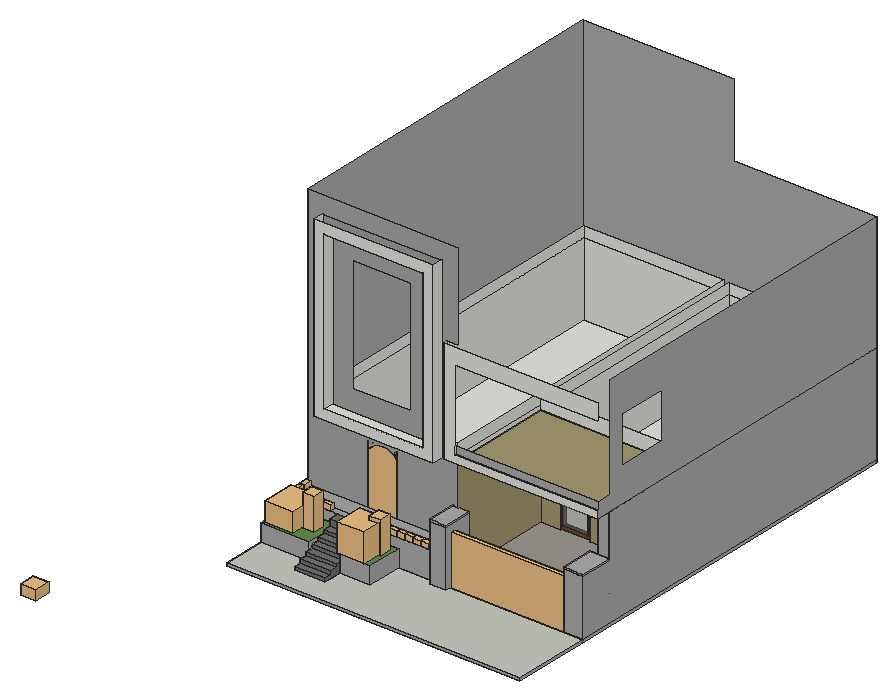
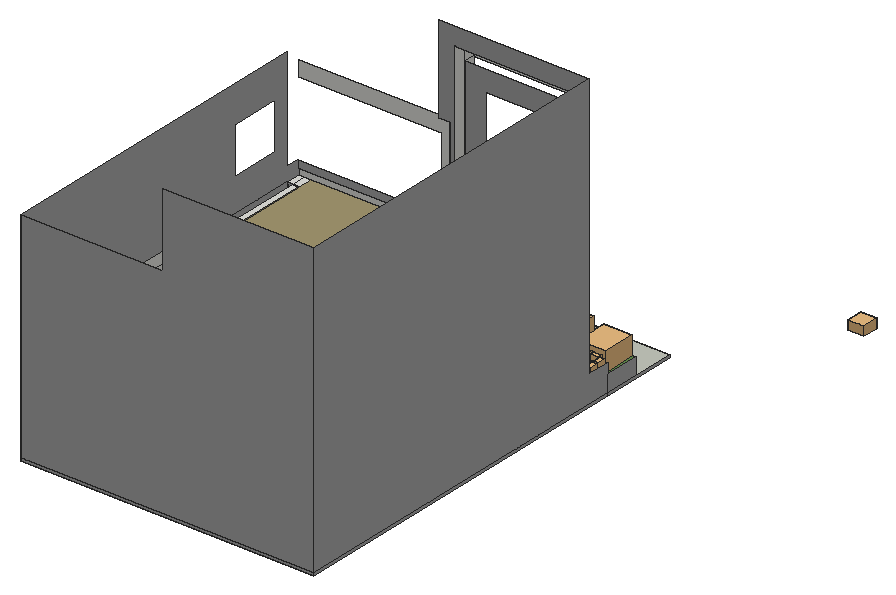
# SketchUp Ruby script. Lengths in inches.
U = 1.inch
M = Sketchup.active_model
def pt(a) = Geom::Point3d.new(a.map { |v| v * U })
def face(e, loops, mat)
  f = e.add_face(loops[0].map { |a| pt(a) })
  loops[1..].each { |l| e.add_face(l.map { |a| pt(a) }).erase! }
  f.material = f.back_material = mat if mat
  f
end
# faces: each face lists its corners as indices into pts; further lists are holes
def faces(e, pts, list, mat = nil) = list.each { |f| face(e, (f[0].is_a?(Array) ? f : [f]).map { |l| l.map { |i| pts[i] } }, mat) }
# xy, xz, yz: faces in a plane at the given z, y or x. An outline is a flat list of corners, or four numbers for a rectangle; further outlines are holes
def ring(l) = l.size == 4 ? [[l[0], l[1]], [l[2], l[1]], [l[2], l[3]], [l[0], l[3]]] : l.each_slice(2).to_a
def flat(e, list, mat, &to3) = list.each { |f| face(e, (f[0].is_a?(Array) ? f : [f]).map { |l| ring(l).map { |u, v| to3.(u, v) } }, mat) }
def xy(e, z, list, mat = nil) = flat(e, list, mat) { |x, y| [x, y, z] }
def xz(e, y, list, mat = nil) = flat(e, list, mat) { |x, z| [x, y, z] }
def yz(e, x, list, mat = nil) = flat(e, list, mat) { |y, z| [x, y, z] }
def lines(e, pts, list) = list.each { |a, b| e.add_line(pt(pts[a]), pt(pts[b])) }
# prism: a flat outline (further loops are holes) pulled along v
def prism(e, loops, v, mat = nil)
  f = face(e, loops, mat); d = Geom::Vector3d.new(v.map { |x| x * U })
  f.pushpull(f.normal.samedirection?(d) ? d.length : -d.length)
end
def box(e, o, s, mat = nil) = prism(e, [[o, [o[0] + s[0], o[1], o[2]], [o[0] + s[0], o[1] + s[1], o[2]], [o[0], o[1] + s[1], o[2]]]], [0, 0, s[2]], mat)
def at(x, y, z, deg = 0) = Geom::Transformation.translation(pt([x, y, z])) * Geom::Transformation.rotation(ORIGIN, Z_AXIS, deg.degrees)
def axes(o, x, y, z) = Geom::Transformation.new([*x, 0, *y, 0, *z, 0, *pt(o).to_a, 1])
def part(name) = M.definitions.add(name)
# library, detail: a bought-in or finely detailed component or shape, given as its bounding box
def library(name, o, s) = part(name).tap { |d| box(d.entities, o, s) }
def detail(e, o, s) = box(e.add_group.entities, o, s)
def put(e, d, t, mat = nil) = e.add_instance(d, t).tap { |i| i.material = mat if mat }
def group(e, t, mat = nil) = e.add_group.tap { |g| g.transformation = t; g.material = mat if mat }.entities
root = M.entities
M.materials.add("[Color M03]").color = [170, 170, 170]
M.materials.add("[Color M05]").color = [114, 114, 114]
M.materials.add("[Granite Tile]").color = [155, 148, 143]
M.materials.add("[Pavers with Grass Herringbone]").color = [197, 201, 190]
M.materials.add("[Stone Vein Gray]").color = [166, 165, 165]
M.materials.add("[Translucent Glass Gray]").color = [128, 128, 128]
M.materials["[Translucent Glass Gray]"].alpha = 0.5
M.materials.add("[Vegetation Grass Artificial]").color = [98, 140, 74]
M.materials.add("[Wood Lumber ButtJoined]").color = [164, 152, 112]
M.materials.add("[Wood Veneer 01]").color = [120, 70, 37]
c1 = library("Plant flower\#1",[15.36,-73.48,0],[25.38,25.65,15.83])
c2 = library("Group\#5",[0,0,0],[194.4375,4,109.5625])
c3 = library("Potted tree",[0,0,0],[18.46,18.88,52.55])
c4 = library("Group3\#1",[-239.85,50.56,0],[44.98,46.36,46.21])
c5 = library("Philodendron 3D",[-30.19,-30.88,0],[62.33,72.62,41.59])
c6 = library("VASINHOS CONCRETO COM SUCULENTAS",[7.69,5.35,0],[7.57,13.06,8.42])
c7 = part("Group\#1")
xy(c7.entities,0,[[0,0,48,9]],"[Wood Veneer 01]")
xy(c7.entities,3.71,[[3.71,0,21.93,9],[26.34,0,44.29,9]],"[Wood Veneer 01]")
xy(c7.entities,80.29,[[3.71,0,21.93,9],[26.34,0,44.29,9]],"[Wood Veneer 01]")
xy(c7.entities,84,[[0,0,48,9]],"[Wood Veneer 01]")
xz(c7.entities,0,[[3.71,3.71,21.93,80.29],[26.34,3.71,44.29,80.29]],"[Translucent Glass Gray]")
xz(c7.entities,0,[[[0,0,48,84],[3.71,3.71,21.93,80.29],[26.34,3.71,44.29,80.29]]],"[Wood Veneer 01]")
xz(c7.entities,9,[[[0,0,48,84],[3.71,3.71,44.29,80.29]],[21.93,3.71,26.34,80.29]],"[Wood Veneer 01]")
yz(c7.entities,0,[[0,0,9,84]],"[Wood Veneer 01]")
yz(c7.entities,3.71,[[0,3.71,9,80.29]],"[Wood Veneer 01]")
yz(c7.entities,21.93,[[0,3.71,9,80.29]],"[Wood Veneer 01]")
yz(c7.entities,26.34,[[0,3.71,9,80.29]],"[Wood Veneer 01]")
yz(c7.entities,44.29,[[0,3.71,9,80.29]],"[Wood Veneer 01]")
yz(c7.entities,48,[[0,0,9,84]],"[Wood Veneer 01]")
xy(root,0,[[4.125,0,484.125,127.875],[4.125,127.875,484.125,727.875]])
xy(root,4,[[83.39,39.19,132.89,51.19],[83.39,51.19,132.89,127.875],[4.125,69.64,83.39,127.875],[4.125,127.875,267.625,127.875,267.625,136.875,484.125,136.875,484.125,727.875,4.125,727.875],[267.625,127.875,475.125,136.875],
  [475.125,127.875,484.125,128.8125],[475.125,128.8125,484.125,136.875]])
xy(root,4,[[4.125,0,484.125,0,484.125,127.875,182.58,127.875,182.58,69.5625,132.89,69.5625,132.89,39.19,83.39,39.19,83.39,69.64,4.125,69.64]],"[Pavers with Grass Herringbone]")
xy(root,4.25,[[241.5,119.1875,267.625,127.875],[452.625,128.8125,475.125,136.875]])
xy(root,4.25,[[267.625,136.875,452.625,136.875,452.625,182.19,465.0625,182.19,465.0625,333.375,331.47,333.375,331.47,339.375,283.47,339.375,283.47,333.375,250.5,333.375,250.5,165.13,267.625,165.13]],"[Granite Tile]")
xy(root,9.5625,[[83.39,39.19,132.89,51.19]],"[Color M05]")
xy(root,15.125,[[83.39,51.19,132.89,63.19]],"[Color M05]")
xy(root,20.6875,[[83.39,63.19,132.89,75.19]],"[Color M05]")
xy(root,26.25,[[83.39,75.19,132.89,87.19]],"[Color M05]")
xy(root,31.8125,[[83.39,87.19,132.89,99.19]],"[Color M05]")
xy(root,31.8125,[[132.89,69.5625,182.58,127.875],[4.125,69.64,83.39,127.875]],"[Vegetation Grass Artificial]")
xy(root,37.375,[[83.39,99.19,132.89,111.19]],"[Color M05]")
xy(root,48,[[13.125,174.8125,241.5,718.875]])
xy(root,48,[[83.39,111.19,132.89,127.875]],"[Color M05]")
xy(root,48,[[4.125,127.875,241.5,127.875,241.5,136.875,13.125,136.875,13.125,165.13,4.125,165.13],[13.125,136.875,241.5,136.875,241.5,165.13,150.96,165.13,150.96,174.8125,102.96,174.8125,102.96,165.13,13.125,165.13]],"[Stone Vein Gray]")
xy(root,55.42,[[383.13,333.375,437.25,339.375]])
xy(root,96,[[452.625,128.8125,484.125,182.19]])
xy(root,99,[[452.625,128.8125,484.125,182.19]],"[Color M03]")
xy(root,99.3125,[[241.5,119.1875,267.625,165.13]],"[Color M03]")
xy(root,111.75,[[283.47,333.375,331.47,339.375]])
xy(root,119.86,[[383.13,333.375,437.25,339.375]])
xy(root,162.49,[[28.46,148.38,223.09,165.13]])
xy(root,168,[[232.4375,157.82,250.5,165.13],[465.0625,157.82,475.125,182.19],[475.125,157.82,484.125,182.19],[465.0625,182.19,475.125,333.375],[483.8125,182.19,484.125,727.875]])
xy(root,168,[[250.5,157.82,465.0625,333.375]],"[Wood Lumber ButtJoined]")
xy(root,178.89,[[44.86,148.38,206.69,165.13]])
xy(root,179.17,[[250.29,157.82,484.125,161.01]])
xz(root,0,[[4.125,0,484.125,4]],"[Color M03]")
xz(root,39.19,[[83.39,4,132.89,9.5625]],"[Color M05]")
xz(root,51.19,[[83.39,9.5625,132.89,15.125]],"[Color M05]")
xz(root,63.19,[[83.39,15.125,132.89,20.6875]],"[Color M05]")
xz(root,69.5625,[[132.89,4,182.58,31.8125]],"[Color M03]")
xz(root,69.64,[[4.125,4,83.39,31.8125]],"[Color M03]")
xz(root,75.19,[[83.39,20.6875,132.89,26.25]],"[Color M05]")
xz(root,87.19,[[83.39,26.25,132.89,31.8125]],"[Color M05]")
xz(root,99.19,[[83.39,31.8125,132.89,37.375]],"[Color M05]")
xz(root,111.19,[[83.39,37.375,132.89,48]],"[Color M05]")
xz(root,119.1875,[[241.5,4.25,267.625,96],[241.5,96,267.625,99.3125]],"[Color M03]")
xz(root,127.875,[[4.125,0,484.125,4],[4.125,4,83.39,31.8125],[83.39,4,132.89,37.375],[132.89,4,182.58,31.8125]])
xz(root,127.875,[[182.58,4,267.625,4,267.625,4.25,241.5,4.25,241.5,48,132.89,48,132.89,31.8125,182.58,31.8125],[4.125,31.8125,83.39,48]],"[Color M03]")
xz(root,128.8125,[[475.125,4,484.125,4,484.125,96,452.625,96,452.625,4.25,475.125,4.25],[452.625,96,484.125,99]],"[Color M03]")
xz(root,136.875,[[267.625,4,475.125,4.25]])
xz(root,148.38,[[[28.46,162.49,223.09,452.06],[44.86,178.89,206.69,435.66]]])
xz(root,157.82,[[232.4375,168,484.125,168,484.125,179.17,250.29,179.17,250.5,192,250.5,312,484.125,312,484.125,337.3125,232.4375,337.3125]])
xz(root,161.01,[[250.29,179.17,484.125,179.17,484.125,192,250.5,192]],"[Color M03]")
xz(root,165.13,[[250.5,4.25,267.625,96],[241.5,96,250.5,99.3125],[250.5,96,267.625,99.3125]])
xz(root,165.13,[[[4.125,48,102.96,48,102.96,132,105.82,135.82,109.27,139.1,113.24,141.76,117.59,143.72,122.2,144.91,126.96,145.3125,131.71,144.91,136.33,143.72,140.68,141.76,144.64,139.1,148.1,135.82,150.96,132,150.96,48,241.5,48,241.5,99.3125,250.5,99.3125,250.5,168,232.4375,168,232.4375,337.3125,250.5,337.3125,250.5,480,4.125,480],[28.46,162.49,223.09,452.06]],[[44.86,178.89,206.69,435.66],[78.82,212.85,172.73,401.7]]],"[Stone Vein Gray]")
xz(root,174.8125,[[13.125,48,13.125,186,241.5,186,241.5,48,150.96,48,150.96,132,148.1,135.82,144.64,139.1,140.68,141.76,136.33,143.72,131.71,144.91,126.96,145.3125,122.2,144.91,117.59,143.72,113.24,141.76,109.27,139.1,105.82,135.82,102.96,132,102.96,48]])
xz(root,182.19,[[452.625,4.25,465.0625,48],[452.625,48,465.0625,96],[452.625,96,465.0625,99],[465.0625,96,483.8125,99],[483.8125,96,484.125,99],
  [483.8125,99,484.125,168]])
xz(root,182.19,[[465.0625,99,483.8125,168]],"[Color M03]")
xz(root,333.375,[[250.5,168,475.125,192]])
xz(root,333.375,[[[250.5,4.25,283.47,4.25,283.47,111.75,331.47,111.75,331.47,4.25,465.0625,4.25,465.0625,168,250.5,168],[383.13,55.42,437.25,119.86]]],"[Wood Lumber ButtJoined]")
xz(root,339.375,[[283.47,4.25,331.47,6.1875],[[250.5,48,250.5,168,475.125,168,475.125,48,331.47,48,331.47,111.75,283.47,111.75,283.47,48],[383.13,55.42,437.25,119.86]],[250.5,168,475.125,186]])
xz(root,718.875,[[13.125,48,241.5,168],[250.5,48,475.125,168],[13.125,168,241.5,186],[250.5,168,475.125,186]])
xz(root,727.875,[[483.8125,48,484.125,168]])
xz(root,727.875,[[4.125,0,484.125,4],[4.125,4,4.125,480,250.5,480,250.5,360,484.125,360,484.125,168,483.8125,168,483.8125,48,484.125,48,484.125,4]],"[Color M03]")
yz(root,4.125,[[0,0,127.875,4],[127.875,0,727.875,4],[69.64,4,127.875,31.8125],[127.875,4,127.875,48,165.13,48,165.13,480,727.875,480,727.875,4]],"[Color M03]")
yz(root,13.125,[[174.8125,48,718.875,168],[174.8125,168,718.875,186]])
yz(root,28.46,[[148.38,162.49,165.13,452.06]])
yz(root,44.86,[[148.38,178.89,165.13,435.66]])
yz(root,83.39,[[69.64,4,69.64,20.6875,75.19,20.6875,75.19,26.25,87.19,26.25,87.19,31.8125,127.875,31.8125,127.875,4]])
yz(root,83.39,[[69.64,20.6875,75.19,20.6875,75.19,26.25,87.19,26.25,87.19,31.8125,69.64,31.8125]],"[Color M03]")
yz(root,83.39,[[39.19,4,39.19,9.5625,51.19,9.5625,51.19,15.125,63.19,15.125,63.19,20.6875,69.64,20.6875,69.64,4],[99.19,31.8125,99.19,37.375,111.19,37.375,111.19,48,127.875,48,127.875,31.8125]],"[Color M05]")
yz(root,102.96,[[165.13,48,174.8125,132]])
yz(root,132.89,[[69.5625,4,127.875,4,127.875,31.8125,87.19,31.8125,87.19,26.25,75.19,26.25,75.19,20.6875,69.5625,20.6875]])
yz(root,132.89,[[69.5625,20.6875,69.5625,31.8125,87.19,31.8125,87.19,26.25,75.19,26.25,75.19,20.6875]],"[Color M03]")
yz(root,132.89,[[39.19,4,69.5625,4,69.5625,20.6875,63.19,20.6875,63.19,15.125,51.19,15.125,51.19,9.5625,39.19,9.5625],[99.19,31.8125,127.875,31.8125,127.875,48,111.19,48,111.19,37.375,99.19,37.375]],"[Color M05]")
yz(root,150.96,[[165.13,48,174.8125,132]])
yz(root,182.58,[[69.5625,4,127.875,31.8125]],"[Color M03]")
yz(root,206.69,[[148.38,178.89,165.13,435.66]])
yz(root,223.09,[[148.38,162.49,165.13,452.06]])
yz(root,232.4375,[[157.82,168,165.13,170],[157.82,170,165.13,337.3125]])
yz(root,241.5,[[174.8125,48,718.875,168],[174.8125,168,718.875,186]])
yz(root,241.5,[[119.1875,4.25,119.1875,99.3125,165.13,99.3125,165.13,48,127.875,48,127.875,4.25]],"[Color M03]")
yz(root,250.5,[[339.375,48,718.875,168],[339.375,168,718.875,186]])
yz(root,250.5,[[165.13,4.25,333.375,168]],"[Wood Lumber ButtJoined]")
yz(root,267.625,[[127.875,4,136.875,4,136.875,4.25,165.13,4.25,165.13,96,119.1875,96,119.1875,4.25,127.875,4.25],[119.1875,96,165.13,99.3125]],"[Color M03]")
yz(root,283.47,[[333.375,4.25,339.375,48],[333.375,48,339.375,111.75]])
yz(root,331.47,[[333.375,4.25,339.375,48],[333.375,48,339.375,111.75]])
yz(root,383.13,[[333.375,55.42,339.375,119.86]])
yz(root,437.25,[[333.375,55.42,339.375,119.86]])
yz(root,452.625,[[128.8125,4.25,182.19,96],[128.8125,96,182.19,99]],"[Color M03]")
yz(root,465.0625,[[182.19,4.25,333.375,168]],"[Wood Lumber ButtJoined]")
yz(root,475.125,[[128.8125,4,136.875,4.25],[339.375,48,718.875,168],[339.375,168,718.875,186]])
yz(root,484.125,[[0,0,127.875,4],[127.875,0,727.875,4],[128.8125,4,727.875,4,727.875,168,182.19,168,182.19,96,128.8125,96],[128.8125,96,182.19,99],[[157.82,168,727.875,168,727.875,360,184.0625,360,184.0625,337.3125,182.19,324,182.19,192,161.01,192,161.01,179.17,157.82,179.17],[207.39,223.41,290.14,299.35]]],"[Color M03]")
p = [[105.82,165.13,135.82],[102.96,165.13,132],[102.96,174.8125,132],[105.82,174.8125,135.82],[150.96,165.13,132],[148.1,165.13,135.82],
  [148.1,174.8125,135.82],[150.96,174.8125,132],[109.27,165.13,139.1],[109.27,174.8125,139.1],[144.64,165.13,139.1],[144.64,174.8125,139.1],
  [113.24,165.13,141.76],[113.24,174.8125,141.76],[140.68,165.13,141.76],[140.68,174.8125,141.76],[117.59,165.13,143.72],[117.59,174.8125,143.72],
  [136.33,165.13,143.72],[136.33,174.8125,143.72],[122.2,165.13,144.91],[122.2,174.8125,144.91],[131.71,165.13,144.91],[131.71,174.8125,144.91],
  [126.96,165.13,145.3125],[126.96,174.8125,145.3125],[250.29,161.01,179.17],[250.5,161.01,192],[250.5,157.82,192],[250.29,157.82,179.17],
  [483.8125,182.19,48],[484.125,182.19,48],[132.89,111.19,31.8125],[83.39,111.19,31.8125],[132.89,99.19,26.25],[83.39,99.19,26.25],
  [132.89,63.19,9.5625],[83.39,63.19,9.5625]]
faces(root,p,[[0,1,2,3],[4,5,6,7],[8,0,3,9],[5,10,11,6],[12,8,9,13],[10,14,15,11],[16,12,13,17],[14,18,19,15],
  [20,16,17,21],[18,22,23,19],[24,20,21,25],[22,24,25,23],[26,27,28,29]])
lines(root,p,[[30,31],[32,33],[34,35],[36,37]])
put(root,c1,at(-170.26,-149.67,0))
put(root,c2,axes([267.625,128.8125,4.25],[0.95146,0,0],[0,1.8,0],[0,0,0.7416]))
g1 = group(root,at(283.47,333.375,6.1875))
xy(g1,0,[[0,0,48,6.9375]],"[Wood Veneer 01]")
xy(g1,4.52,[[3.62,0,44.38,0.9375],[3.62,0.9375,44.38,6.9375]],"[Wood Veneer 01]")
xy(g1,100.48,[[3.62,0,44.38,0.9375],[3.62,0.9375,44.38,6.9375]],"[Wood Veneer 01]")
xy(g1,105,[[0,0,48,6.9375]],"[Wood Veneer 01]")
xz(g1,0,[[[0,0,48,105],[3.62,4.52,44.38,100.48]]],"[Wood Veneer 01]")
xz(g1,0.9375,[[3.62,4.52,44.38,100.48]],"[Translucent Glass Gray]")
xz(g1,6.9375,[[[0,0,48,105],[3.62,4.52,44.38,100.48]]],"[Wood Veneer 01]")
yz(g1,0,[[0,0,6.9375,105]],"[Wood Veneer 01]")
yz(g1,3.62,[[0,4.52,0.9375,100.48],[0.9375,4.52,6.9375,100.48]],"[Wood Veneer 01]")
yz(g1,44.38,[[0,4.52,0.9375,100.48],[0.9375,4.52,6.9375,100.48]],"[Wood Veneer 01]")
yz(g1,48,[[0,0,6.9375,105]],"[Wood Veneer 01]")
put(root,c3,at(53.32,93.3,31.8125))
put(root,c3,at(158.13,98.86,31.8125))
put(root,c4,at(368.11,19.01,31.8125))
put(root,c5,axes([30.01,96.57,32.89],[0.75,0,0],[0,0.75,0],[0,0,0.75]))
g2 = group(root,at(102.96,165.13,48))
detail(g2,[0,0,0],[48,8.25,97.44])
put(root,c6,at(-3.14,143.71,48))
put(root,c6,at(-3.14,127.9,48))
put(root,c6,at(8.3125,143.13,48,-90))
put(root,c6,at(24.625,143.13,48,-90))
put(root,c6,at(39.1875,143.13,48,-90))
put(root,c6,at(53.0625,143.13,48,-90))
put(root,c6,at(131.41,143.13,48,-90))
put(root,c6,at(146.23,143.13,48,-90))
put(root,c6,at(161.48,143.13,48,-90))
put(root,c6,at(174.79,143.13,48,-90))
put(root,c6,at(187.91,143.13,48,-90))
put(root,c6,at(201.04,143.13,48,-90))
put(root,c6,at(213.91,143.13,48,-90))
put(root,c7,axes([383.37,333.375,55.42],[1.12254,0,0],[0,1,0],[0,0,0.76711]))
